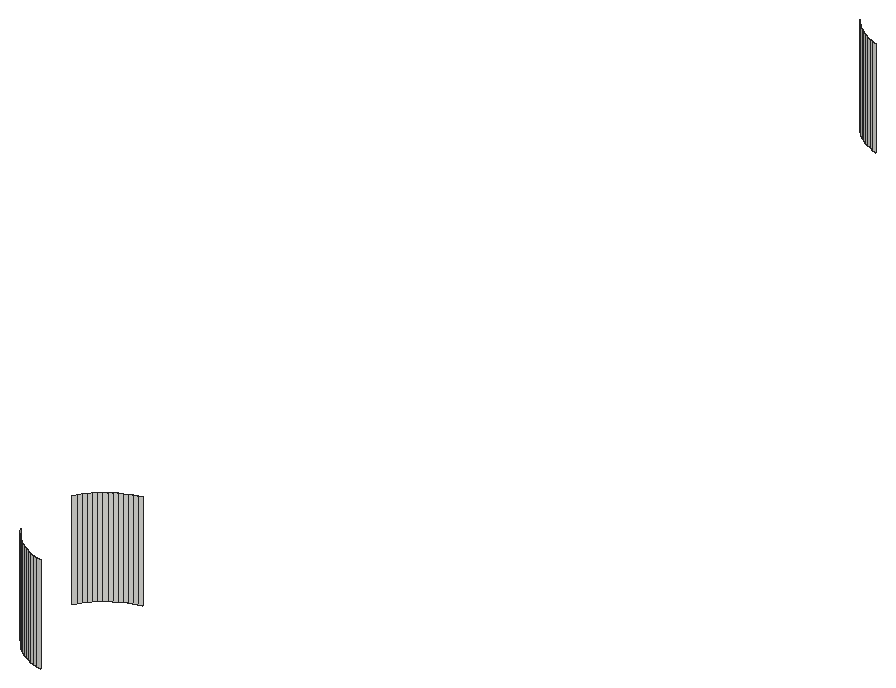
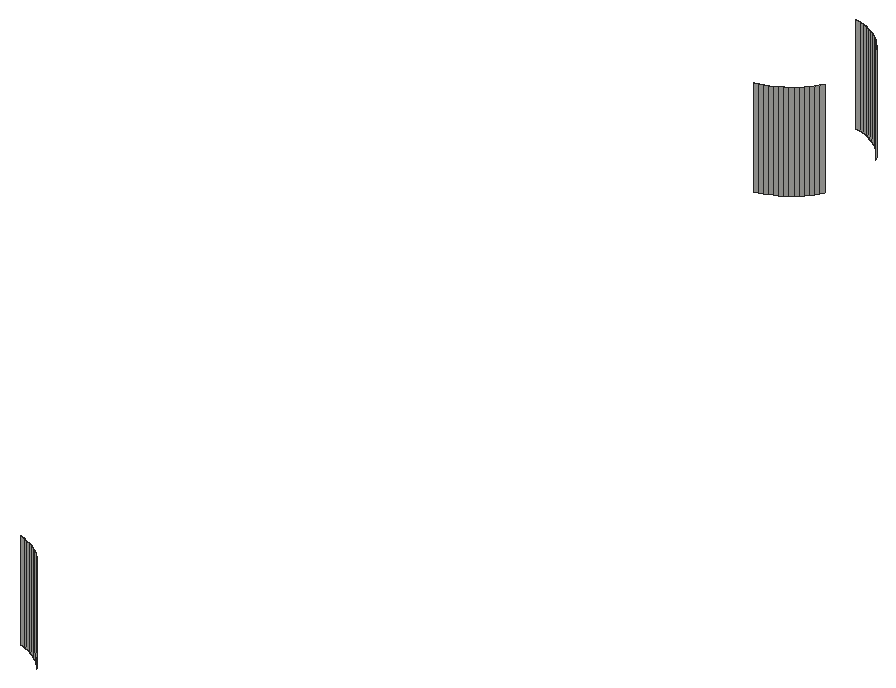
# SketchUp Ruby script. Lengths in millimetres.
U = 1.mm
M = Sketchup.active_model
def pt(a) = Geom::Point3d.new(a.map { |v| v * U })
def face(e, loops, mat)
  f = e.add_face(loops[0].map { |a| pt(a) })
  loops[1..].each { |l| e.add_face(l.map { |a| pt(a) }).erase! }
  f.material = f.back_material = mat if mat
  f
end
# faces: each face lists its corners as indices into pts; further lists are holes
def faces(e, pts, list, mat = nil) = list.each { |f| face(e, (f[0].is_a?(Array) ? f : [f]).map { |l| l.map { |i| pts[i] } }, mat) }
# xy, xz, yz: faces in a plane at the given z, y or x. An outline is a flat list of corners, or four numbers for a rectangle; further outlines are holes
def ring(l) = l.size == 4 ? [[l[0], l[1]], [l[2], l[1]], [l[2], l[3]], [l[0], l[3]]] : l.each_slice(2).to_a
def flat(e, list, mat, &to3) = list.each { |f| face(e, (f[0].is_a?(Array) ? f : [f]).map { |l| ring(l).map { |u, v| to3.(u, v) } }, mat) }
def xy(e, z, list, mat = nil) = flat(e, list, mat) { |x, y| [x, y, z] }
def xz(e, y, list, mat = nil) = flat(e, list, mat) { |x, z| [x, y, z] }
def yz(e, x, list, mat = nil) = flat(e, list, mat) { |y, z| [x, y, z] }
def lines(e, pts, list) = list.each { |a, b| e.add_line(pt(pts[a]), pt(pts[b])) }
# prism: a flat outline (further loops are holes) pulled along v
def prism(e, loops, v, mat = nil)
  f = face(e, loops, mat); d = Geom::Vector3d.new(v.map { |x| x * U })
  f.pushpull(f.normal.samedirection?(d) ? d.length : -d.length)
end
def box(e, o, s, mat = nil) = prism(e, [[o, [o[0] + s[0], o[1], o[2]], [o[0] + s[0], o[1] + s[1], o[2]], [o[0], o[1] + s[1], o[2]]]], [0, 0, s[2]], mat)
def at(x, y, z, deg = 0) = Geom::Transformation.translation(pt([x, y, z])) * Geom::Transformation.rotation(ORIGIN, Z_AXIS, deg.degrees)
def axes(o, x, y, z) = Geom::Transformation.new([*x, 0, *y, 0, *z, 0, *pt(o).to_a, 1])
def part(name) = M.definitions.add(name)
# library, detail: a bought-in or finely detailed component or shape, given as its bounding box
def library(name, o, s) = part(name).tap { |d| box(d.entities, o, s) }
def detail(e, o, s) = box(e.add_group.entities, o, s)
def put(e, d, t, mat = nil) = e.add_instance(d, t).tap { |i| i.material = mat if mat }
def group(e, t, mat = nil) = e.add_group.tap { |g| g.transformation = t; g.material = mat if mat }.entities
root = M.entities
p = [[3469.6,997.1,2718.2],[3469.6,997.1,2794],[3472.7,996.4,2794],[3472.7,996.4,2718.2],[3466.5,998,2718.2],[3466.5,998,2794],
  [3463.5,999,2718.2],[3463.5,999,2794],[3460.6,1000.3,2718.2],[3460.6,1000.3,2794],[3457.7,1001.8,2718.2],[3457.7,1001.8,2794],
  [3455,1003.4,2718.2],[3455,1003.4,2794],[3452.3,1005.2,2718.2],[3452.3,1005.2,2794],[3449.8,1007.1,2718.2],[3449.8,1007.1,2794],
  [3447.4,1009.2,2718.2],[3447.4,1009.2,2794],[3445.2,1011.5,2718.2],[3445.2,1011.5,2794],[3443.1,1013.9,2718.2],[3443.1,1013.9,2794],
  [3441.1,1016.4,2718.2],[3441.1,1016.4,2794],[3439.3,1019,2718.2],[3439.3,1019,2794],[3439.3,1073.5,2718.2],[3439.3,1073.5,2794],
  [3437.7,1070.7,2794],[3437.7,1070.7,2718.2],[3441.1,1076.1,2718.2],[3441.1,1076.1,2794],[3443.1,1078.6,2718.2],[3443.1,1078.6,2794],
  [3445.2,1081,2718.2],[3445.2,1081,2794],[3447.4,1083.3,2718.2],[3447.4,1083.3,2794],[3449.8,1085.4,2718.2],[3449.8,1085.4,2794],
  [3452.3,1087.4,2718.2],[3452.3,1087.4,2794],[3455,1089.2,2718.2],[3455,1089.2,2794],[3457.7,1090.8,2718.2],[3457.7,1090.8,2794],
  [3460.6,1092.2,2718.2],[3460.6,1092.2,2794],[3463.5,1093.5,2718.2],[3463.5,1093.5,2794],[3466.5,1094.6,2718.2],[3466.5,1094.6,2794],
  [3469.6,1095.5,2718.2],[3469.6,1095.5,2794],[3472.7,1096.2,2718.2],[3472.7,1096.2,2794],[3466.5,1815.6,2718.2],[3466.5,1815.6,2794],
  [3469.6,1814.7,2794],[3469.6,1814.7,2718.2],[3463.5,1816.7,2718.2],[3463.5,1816.7,2794],[3460.6,1818,2718.2],[3460.6,1818,2794],
  [3457.7,1819.4,2718.2],[3457.7,1819.4,2794],[3455,1821,2718.2],[3455,1821,2794],[3452.3,1822.8,2718.2],[3452.3,1822.8,2794],
  [3449.8,1824.8,2718.2],[3449.8,1824.8,2794],[3447.4,1826.9,2718.2],[3447.4,1826.9,2794],[3445.2,1829.2,2718.2],[3445.2,1829.2,2794],
  [3443.1,1831.6,2718.2],[3443.1,1831.6,2794]]
faces(root,p,[[0,1,2,3],[4,5,1,0],[6,7,5,4],[8,9,7,6],[10,11,9,8],[12,13,11,10],[14,15,13,12],[16,17,15,14],
  [18,19,17,16],[20,21,19,18],[22,23,21,20],[24,25,23,22],[26,27,25,24],[28,29,30,31],[32,33,29,28],[34,35,33,32],
  [36,37,35,34],[38,39,37,36],[40,41,39,38],[42,43,41,40],[44,45,43,42],[46,47,45,44],[48,49,47,46],[50,51,49,48],
  [52,53,51,50],[54,55,53,52],[56,57,55,54],[58,59,60,61],[62,63,59,58],[64,65,63,62],[66,67,65,64],[68,69,67,66],
  [70,71,69,68],[72,73,71,70],[74,75,73,72],[76,77,75,74],[78,79,77,76]])
